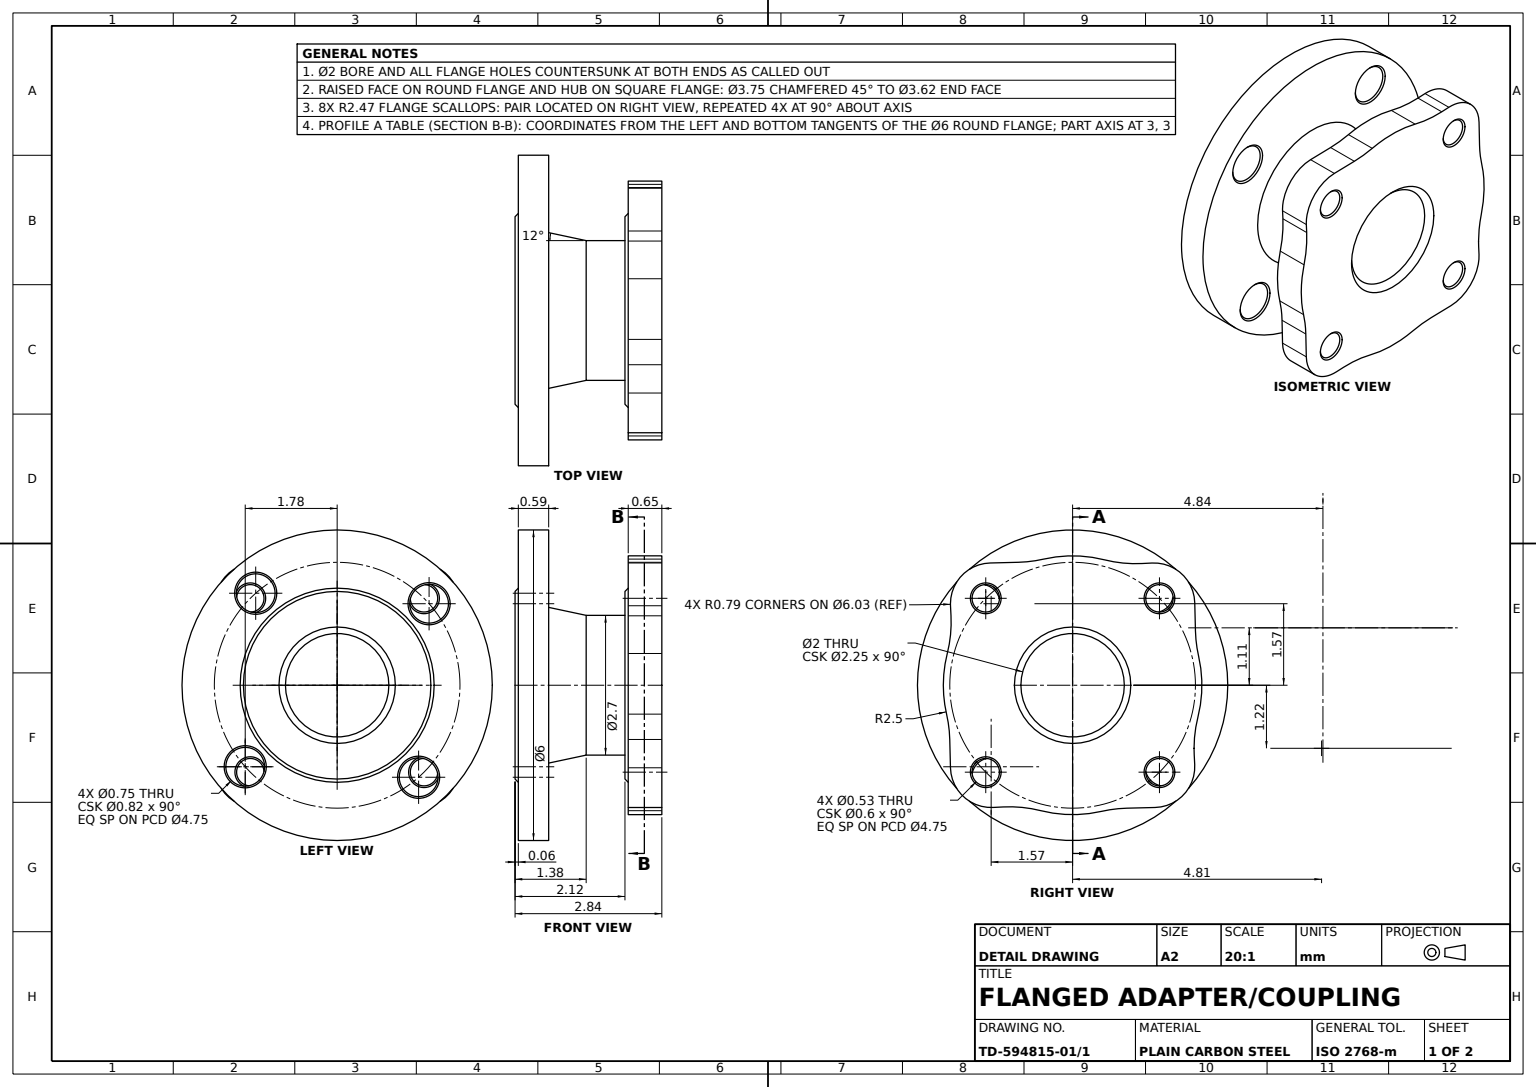
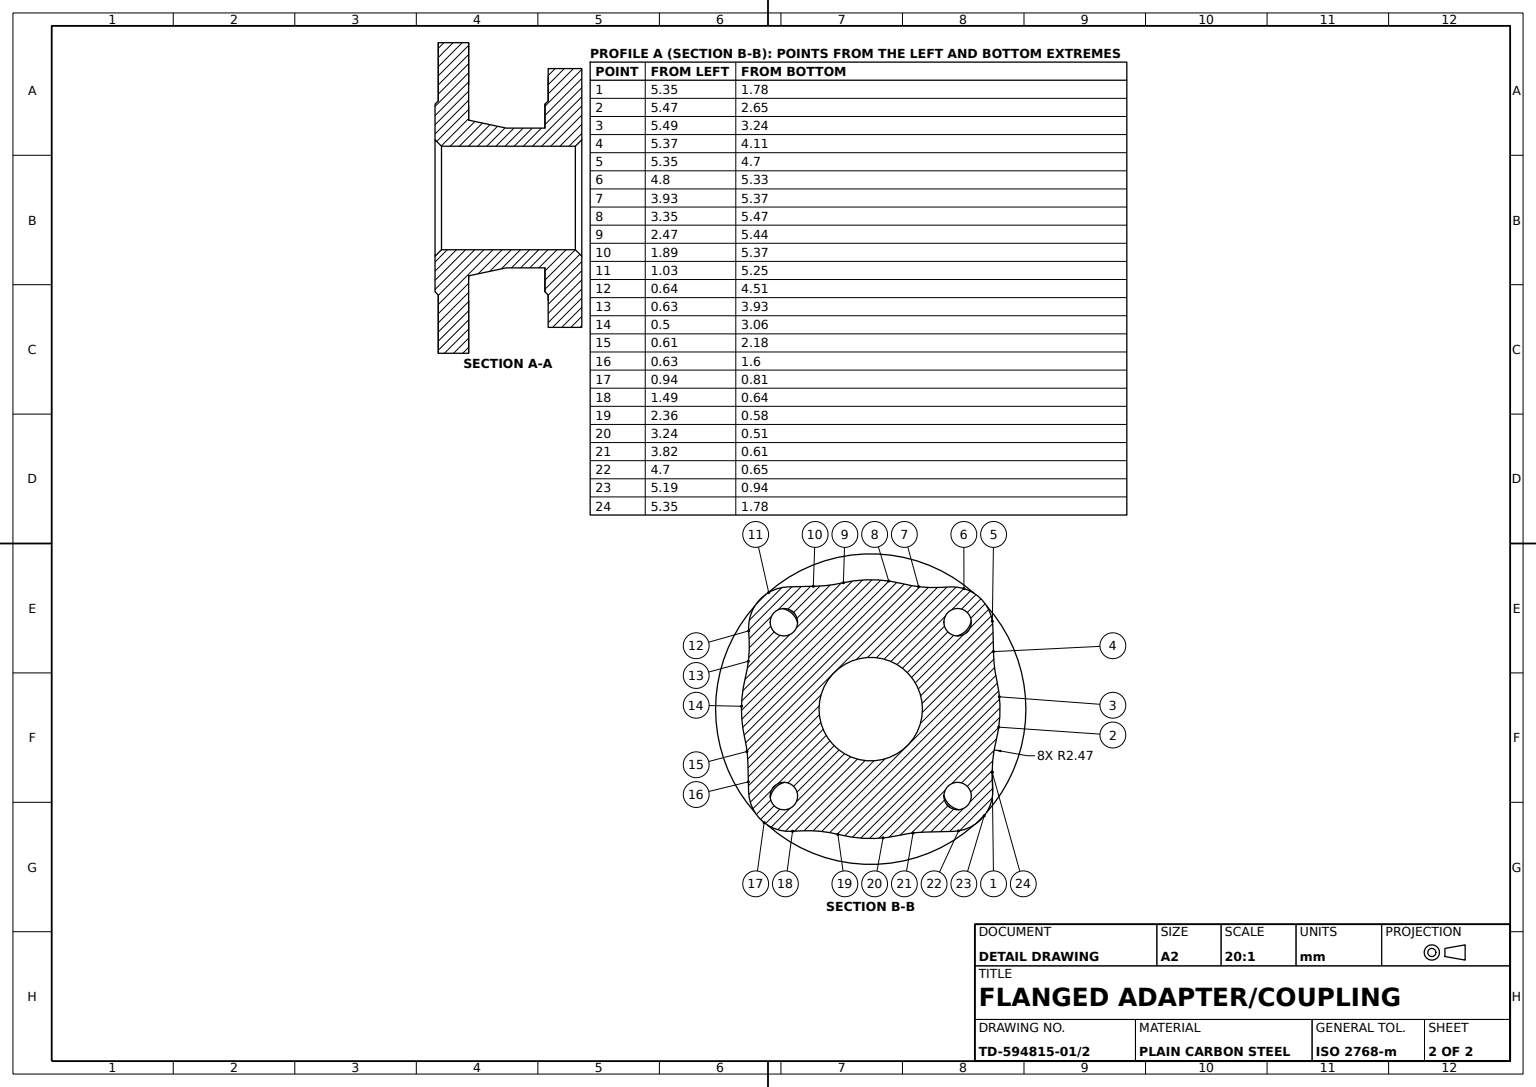
solid
v1 (2.838,0.558304,-2.436862)
v2 (2.838,1.047699,-2.375349)
e1 v1 v2 CIRCLE(AX(P(2.838,1.108969,-4.840385),D(-1,0,0),D(0,0,-1)),2.465797)
v3 (2.188,0.558304,-2.436862)
e2 v1 v3 LINE
v4 (2.188,1.047699,-2.375349)
e3 v3 v4 CIRCLE(AX(P(2.188,1.108969,-4.840385),D(-1,0,0),D(0,0,-1)),2.465797)
e4 v2 v4 LINE
face CYL(AX(P(2.838,1.108969,-4.840385),D(-1,0,0),D(0,0,1)),2.465797) rev [-e1 e2 e3 -e4]
v5 (0.6175,-1.777639,1.95)
v6 (0.65,-1.777639,1.9825)
e5 v5 v6 LINE
v7 (0.65,-1.777639,1.1675)
e6 v7 v6 CIRCLE(AX(P(0.65,-1.777639,1.575),D(-1,0,0),D(0,0,1)),0.4075)
v8 (0.6175,-1.777639,1.2)
e7 v8 v7 LINE
e8 v5 v8 CIRCLE(AX(P(0.6175,-1.777639,1.575),D(1,0,0),D(0,0,1)),0.375)
face CONE(AX(P(0.65,-1.777639,1.575),D(1,0,0),D(0,0,-1)),0.4075,0.785398163) rev [e5 -e6 -e7 -e8]
v9 (2.188,0,1.875)
v10 (2.188,0,-1.875)
e9 v9 v10 CIRCLE(AX(P(2.188,0,0),D(-1,0,0),D(0,0,1)),1.875)
v11 (2.125,0,-1.812)
e10 v11 v10 LINE
v12 (2.125,0,1.812)
e11 v12 v11 CIRCLE(AX(P(2.125,0,0),D(-1,0,0),D(0,0,1)),1.812)
e12 v12 v9 LINE
face CONE(AX(P(2.188,0,0),D(1,0,0),D(0,0,-1)),1.875,0.785398163) [e9 -e10 -e11 e12]
v13 (2.8055,-1.679379,1.414379)
v14 (2.8055,-1.679379,1.944379)
e13 v13 v14 CIRCLE(AX(P(2.8055,-1.679379,1.679379),D(1,0,0),D(0,0,-1)),0.265)
v15 (2.838,-1.679379,1.381879)
e14 v13 v15 LINE
v16 (2.838,-1.679379,1.976879)
e15 v16 v15 CIRCLE(AX(P(2.838,-1.679379,1.679379),D(-1,0,0),D(0,0,-1)),0.2975)
e16 v14 v16 LINE
face CONE(AX(P(2.8055,-1.679379,1.679379),D(1,0,0),D(0,0,-1)),0.265,0.785398163) rev [-e13 e14 -e15 -e16]
v17 (2.2205,-1.679379,-1.944379)
v18 (2.2205,-1.679379,-1.414379)
e17 v17 v18 CIRCLE(AX(P(2.2205,-1.679379,-1.679379),D(-1,0,0),D(0,0,-1)),0.265)
v19 (2.188,-1.679379,-1.976879)
e18 v17 v19 LINE
v20 (2.188,-1.679379,-1.381879)
e19 v20 v19 CIRCLE(AX(P(2.188,-1.679379,-1.679379),D(1,0,0),D(0,0,-1)),0.2975)
e20 v18 v20 LINE
face CONE(AX(P(2.188,-1.679379,-1.679379),D(-1,0,0),D(0,0,1)),0.2975,0.785398163) rev [-e17 e18 -e19 -e20]
v21 (0.0955,-1.777639,1.2)
v22 (0.063,-1.777639,1.1675)
e21 v21 v22 LINE
v23 (0.063,-1.777639,1.9825)
e22 v23 v22 CIRCLE(AX(P(0.063,-1.777639,1.575),D(1,0,0),D(0,0,-1)),0.4075)
v24 (0.0955,-1.777639,1.95)
e23 v24 v23 LINE
e24 v21 v24 CIRCLE(AX(P(0.0955,-1.777639,1.575),D(-1,0,0),D(0,0,-1)),0.375)
face CONE(AX(P(0.0955,-1.777639,1.575),D(-1,0,0),D(0,0,1)),0.375,0.785398163) rev [e21 -e22 -e23 -e24]
v25 (0.6175,-1.575,-1.402639)
v26 (0.65,-1.575,-1.370139)
e25 v25 v26 LINE
v27 (0.65,-1.575,-2.185139)
e26 v27 v26 CIRCLE(AX(P(0.65,-1.575,-1.777639),D(-1,0,0),D(0,0,1)),0.4075)
v28 (0.6175,-1.575,-2.152639)
e27 v28 v27 LINE
e28 v25 v28 CIRCLE(AX(P(0.6175,-1.575,-1.777639),D(1,0,0),D(0,0,1)),0.375)
face CONE(AX(P(0.65,-1.575,-1.777639),D(1,0,0),D(0,0,-1)),0.4075,0.785398163) rev [e25 -e26 -e27 -e28]
v29 (2.8055,1.679379,-1.414379)
v30 (2.838,1.679379,-1.381879)
e29 v29 v30 LINE
v31 (2.8055,1.679379,-1.944379)
e30 v31 v29 CIRCLE(AX(P(2.8055,1.679379,-1.679379),D(1,0,0),D(0,0,-1)),0.265)
v32 (2.838,1.679379,-1.976879)
e31 v31 v32 LINE
e32 v30 v32 CIRCLE(AX(P(2.838,1.679379,-1.679379),D(-1,0,0),D(0,0,-1)),0.2975)
face CONE(AX(P(2.8055,1.679379,-1.679379),D(1,0,0),D(0,0,-1)),0.265,0.785398163) rev [-e29 -e30 e31 -e32]
e33 v11 v12 CIRCLE(AX(P(2.125,0,0),D(-1,0,0),D(0,0,1)),1.812)
v33 (2.125,0,1.35)
v34 (2.125,0,-1.35)
e34 v33 v34 CIRCLE(AX(P(2.125,0,0),D(-1,0,0),D(0,0,1)),1.35)
e35 v34 v33 CIRCLE(AX(P(2.125,0,0),D(-1,0,0),D(0,0,1)),1.35)
face PLANE(AX(P(2.125,1.35,0),D(1,0,0),D(0,0,-1))) rev [e11 e33] [-e34 -e35]
v35 (2.713,0,1)
v36 (2.713,0,-1)
e36 v35 v36 CIRCLE(AX(P(2.713,0,0),D(1,0,0),D(0,0,-1)),1)
v37 (0.125,0,-1)
e37 v36 v37 LINE
v38 (0.125,0,1)
e38 v37 v38 CIRCLE(AX(P(0.125,0,0),D(-1,0,0),D(0,0,-1)),1)
e39 v35 v38 LINE
face CYL(AX(P(0,0,0),D(-1,0,0),D(0,0,1)),1) rev [e36 e37 e38 -e39]
v39 (1.375,0,-1.35)
v40 (1.375,0,1.35)
e40 v39 v40 CIRCLE(AX(P(1.375,0,0),D(-1,0,0),D(0,0,1)),1.35)
e41 v34 v39 LINE
e42 v33 v40 LINE
face CYL(AX(P(0,0,0),D(-1,0,0),D(0,0,1)),1.35) [-e40 -e41 e35 e42]
v41 (2.838,-2.375349,-1.047699)
v42 (2.188,-2.375349,-1.047699)
e43 v41 v42 LINE
v43 (2.188,-2.361757,-1.594555)
e44 v42 v43 LINE
v44 (2.838,-2.361757,-1.594555)
e45 v44 v43 LINE
e46 v41 v44 LINE
face PLANE(AX(P(2.838,-2.361757,-1.594555),D(0,0.999691244,0.024847874),D(0,-0.024847874,0.999691244))) rev [e43 e44 -e45 -e46]
v45 (0.6175,1.575,2.152639)
v46 (0.0955,1.575,2.152639)
e47 v45 v46 LINE
v47 (0.6175,1.575,1.402639)
e48 v45 v47 CIRCLE(AX(P(0.6175,1.575,1.777639),D(1,0,0),D(0,0,1)),0.375)
v48 (0.0955,1.575,1.402639)
e49 v47 v48 LINE
e50 v48 v46 CIRCLE(AX(P(0.0955,1.575,1.777639),D(-1,0,0),D(0,0,-1)),0.375)
face CYL(AX(P(0.713,1.575,1.777639),D(-1,0,0),D(0,0,1)),0.375) rev [-e47 e48 e49 e50]
e51 v8 v21 LINE
e52 v8 v5 CIRCLE(AX(P(0.6175,-1.777639,1.575),D(1,0,0),D(0,0,1)),0.375)
e53 v5 v24 LINE
e54 v24 v21 CIRCLE(AX(P(0.0955,-1.777639,1.575),D(-1,0,0),D(0,0,-1)),0.375)
face CYL(AX(P(0.713,-1.777639,1.575),D(-1,0,0),D(0,0,1)),0.375) rev [-e51 e52 e53 e54]
v49 (0.65,0,3)
v50 (0.65,0,-3)
e55 v49 v50 CIRCLE(AX(P(0.65,0,0),D(-1,0,0),D(0,0,1)),3)
v51 (0.063,0,-3)
e56 v50 v51 LINE
v52 (0.063,0,3)
e57 v52 v51 CIRCLE(AX(P(0.063,0,0),D(-1,0,0),D(0,0,1)),3)
e58 v49 v52 LINE
face CYL(AX(P(0,0,0),D(-1,0,0),D(0,0,1)),3) [e55 e56 -e57 -e58]
v53 (2.188,-2.436862,-0.558304)
e59 v53 v42 CIRCLE(AX(P(2.188,-4.840385,-1.108969),D(-1,0,0),D(0,0,-1)),2.465797)
v54 (2.838,-2.436862,-0.558304)
e60 v54 v41 CIRCLE(AX(P(2.838,-4.840385,-1.108969),D(-1,0,0),D(0,0,-1)),2.465797)
e61 v54 v53 LINE
face CYL(AX(P(2.838,-4.840385,-1.108969),D(-1,0,0),D(0,0,1)),2.465797) rev [e59 -e43 -e60 e61]
e62 v10 v9 CIRCLE(AX(P(2.188,0,0),D(-1,0,0),D(0,0,1)),1.875)
face CONE(AX(P(2.188,0,0),D(1,0,0),D(0,0,-1)),1.875,0.785398163) [e10 e62 -e12 -e33]
v55 (2.838,0,1.125)
e63 v35 v55 LINE
v56 (2.838,0,-1.125)
e64 v56 v55 CIRCLE(AX(P(2.838,0,0),D(-1,0,0),D(0,0,-1)),1.125)
e65 v36 v56 LINE
face CONE(AX(P(2.713,0,0),D(1,0,0),D(0,0,-1)),1,0.785398163) rev [-e36 e63 -e64 -e65]
v57 (0.063,1.777639,-1.9825)
v58 (0.063,1.777639,-1.1675)
e66 v57 v58 CIRCLE(AX(P(0.063,1.777639,-1.575),D(1,0,0),D(0,0,-1)),0.4075)
v59 (0.0955,1.777639,-1.95)
e67 v59 v57 LINE
v60 (0.0955,1.777639,-1.2)
e68 v60 v59 CIRCLE(AX(P(0.0955,1.777639,-1.575),D(-1,0,0),D(0,0,-1)),0.375)
e69 v60 v58 LINE
face CONE(AX(P(0.0955,1.777639,-1.575),D(-1,0,0),D(0,0,1)),0.375,0.785398163) rev [-e66 -e67 -e68 e69]
v61 (2.2205,1.679379,1.414379)
v62 (2.2205,1.679379,1.944379)
e70 v61 v62 CIRCLE(AX(P(2.2205,1.679379,1.679379),D(-1,0,0),D(0,0,-1)),0.265)
v63 (2.188,1.679379,1.381879)
e71 v61 v63 LINE
v64 (2.188,1.679379,1.976879)
e72 v64 v63 CIRCLE(AX(P(2.188,1.679379,1.679379),D(1,0,0),D(0,0,-1)),0.2975)
e73 v62 v64 LINE
face CONE(AX(P(2.188,1.679379,1.679379),D(-1,0,0),D(0,0,1)),0.2975,0.785398163) rev [-e70 e71 -e72 -e73]
v65 (0.063,1.575,2.185139)
e74 v46 v65 LINE
v66 (0.063,1.575,1.370139)
e75 v66 v65 CIRCLE(AX(P(0.063,1.575,1.777639),D(1,0,0),D(0,0,-1)),0.4075)
e76 v48 v66 LINE
e77 v46 v48 CIRCLE(AX(P(0.0955,1.575,1.777639),D(-1,0,0),D(0,0,-1)),0.375)
face CONE(AX(P(0.0955,1.575,1.777639),D(-1,0,0),D(0,0,1)),0.375,0.785398163) rev [e74 -e75 -e76 -e77]
e78 v62 v61 CIRCLE(AX(P(2.2205,1.679379,1.679379),D(-1,0,0),D(0,0,-1)),0.265)
e79 v63 v64 CIRCLE(AX(P(2.188,1.679379,1.679379),D(1,0,0),D(0,0,-1)),0.2975)
face CONE(AX(P(2.188,1.679379,1.679379),D(-1,0,0),D(0,0,1)),0.2975,0.785398163) rev [-e78 e73 -e79 -e71]
v67 (2.2205,1.679379,-1.944379)
e80 v31 v67 LINE
v68 (2.2205,1.679379,-1.414379)
e81 v67 v68 CIRCLE(AX(P(2.2205,1.679379,-1.679379),D(-1,0,0),D(0,0,-1)),0.265)
e82 v29 v68 LINE
e83 v29 v31 CIRCLE(AX(P(2.8055,1.679379,-1.679379),D(1,0,0),D(0,0,-1)),0.265)
face CYL(AX(P(2.838,1.679379,-1.679379),D(-1,0,0),D(0,0,1)),0.265) rev [e80 e81 -e82 e83]
v69 (2.188,1.679379,-1.381879)
e84 v68 v69 LINE
v70 (2.188,1.679379,-1.976879)
e85 v70 v69 CIRCLE(AX(P(2.188,1.679379,-1.679379),D(1,0,0),D(0,0,-1)),0.2975)
e86 v67 v70 LINE
e87 v68 v67 CIRCLE(AX(P(2.2205,1.679379,-1.679379),D(-1,0,0),D(0,0,-1)),0.265)
face CONE(AX(P(2.188,1.679379,-1.679379),D(-1,0,0),D(0,0,1)),0.2975,0.785398163) rev [e84 -e85 -e86 -e87]
v71 (0,0,1.125)
e88 v38 v71 LINE
v72 (0,0,-1.125)
e89 v72 v71 CIRCLE(AX(P(0,0,0),D(1,0,0),D(0,0,-1)),1.125)
e90 v37 v72 LINE
e91 v38 v37 CIRCLE(AX(P(0.125,0,0),D(-1,0,0),D(0,0,-1)),1)
face CONE(AX(P(0.125,0,0),D(-1,0,0),D(0,0,1)),1,0.785398163) rev [e88 -e89 -e90 -e91]
v73 (2.8055,-1.679379,-1.414379)
e92 v73 v18 LINE
e93 v18 v17 CIRCLE(AX(P(2.2205,-1.679379,-1.679379),D(-1,0,0),D(0,0,-1)),0.265)
v74 (2.8055,-1.679379,-1.944379)
e94 v74 v17 LINE
e95 v74 v73 CIRCLE(AX(P(2.8055,-1.679379,-1.679379),D(1,0,0),D(0,0,-1)),0.265)
face CYL(AX(P(2.838,-1.679379,-1.679379),D(-1,0,0),D(0,0,1)),0.265) rev [e92 e93 -e94 e95]
e96 v69 v70 CIRCLE(AX(P(2.188,1.679379,-1.679379),D(1,0,0),D(0,0,-1)),0.2975)
v75 (2.188,-1.679379,1.381879)
v76 (2.188,-1.679379,1.976879)
e97 v75 v76 CIRCLE(AX(P(2.188,-1.679379,1.679379),D(1,0,0),D(0,0,-1)),0.2975)
e98 v76 v75 CIRCLE(AX(P(2.188,-1.679379,1.679379),D(1,0,0),D(0,0,-1)),0.2975)
e99 v19 v20 CIRCLE(AX(P(2.188,-1.679379,-1.679379),D(1,0,0),D(0,0,-1)),0.2975)
v77 (2.188,-1.218309,-2.348231)
v78 (2.188,-0.61335,-2.423593)
e100 v77 v78 CIRCLE(AX(P(2.188,-1.218309,-4.814028),D(-1,0,0),D(0,0,1)),2.465797)
v79 (2.188,-1.341424,-2.351306)
e101 v79 v77 CIRCLE(AX(P(2.188,-1.218309,-4.814028),D(-1,0,0),D(0,0,1)),2.465797)
v80 (2.188,-1.535706,-2.361018)
e102 v80 v79 LINE
e103 v43 v80 CIRCLE(AX(P(2.188,-1.575,-1.575),D(1,0,0),D(0,0,-1)),0.787)
v81 (2.188,-2.423593,0.61335)
e104 v81 v53 CIRCLE(AX(P(2.188,0,0),D(1,0,0),D(0,0,-1)),2.5)
v82 (2.188,-2.351306,1.341424)
e105 v82 v81 CIRCLE(AX(P(2.188,-4.814028,1.218309),D(-1,0,0),D(0,0,1)),2.465797)
v83 (2.188,-2.361018,1.535706)
e106 v83 v82 LINE
v84 (2.188,-1.594555,2.361757)
e107 v84 v83 CIRCLE(AX(P(2.188,-1.575,1.575),D(1,0,0),D(0,0,-1)),0.787)
v85 (2.188,-1.047699,2.375349)
e108 v85 v84 LINE
v86 (2.188,-0.558304,2.436862)
e109 v86 v85 CIRCLE(AX(P(2.188,-1.108969,4.840385),D(-1,0,0),D(0,0,-1)),2.465797)
v87 (2.188,0,2.5)
e110 v87 v86 CIRCLE(AX(P(2.188,0,0),D(1,0,0),D(0,0,-1)),2.5)
v88 (2.188,0.61335,2.423593)
e111 v88 v87 CIRCLE(AX(P(2.188,0,0),D(1,0,0),D(0,0,-1)),2.5)
v89 (2.188,1.341424,2.351306)
e112 v89 v88 CIRCLE(AX(P(2.188,1.218309,4.814028),D(-1,0,0),D(0,0,1)),2.465797)
v90 (2.188,1.535706,2.361018)
e113 v90 v89 LINE
v91 (2.188,1.575,2.362)
e114 v91 v90 CIRCLE(AX(P(2.188,1.575,1.575),D(1,0,0),D(0,0,-1)),0.787)
v92 (2.188,2.361757,1.594555)
e115 v92 v91 CIRCLE(AX(P(2.188,1.575,1.575),D(1,0,0),D(0,0,-1)),0.787)
v93 (2.188,2.375349,1.047699)
e116 v93 v92 LINE
v94 (2.188,2.436862,0.558304)
e117 v94 v93 CIRCLE(AX(P(2.188,4.840385,1.108969),D(-1,0,0),D(0,0,1)),2.465797)
v95 (2.188,2.423593,-0.61335)
e118 v95 v94 CIRCLE(AX(P(2.188,0,0),D(1,0,0),D(0,0,-1)),2.5)
v96 (2.188,2.351306,-1.341424)
e119 v96 v95 CIRCLE(AX(P(2.188,4.814028,-1.218309),D(-1,0,0),D(0,0,1)),2.465797)
v97 (2.188,2.361018,-1.535706)
e120 v97 v96 LINE
v98 (2.188,1.594555,-2.361757)
e121 v98 v97 CIRCLE(AX(P(2.188,1.575,-1.575),D(1,0,0),D(0,0,-1)),0.787)
e122 v4 v98 LINE
e123 v78 v3 CIRCLE(AX(P(2.188,0,0),D(1,0,0),D(0,0,-1)),2.5)
face PLANE(AX(P(2.188,1.575,1.575),D(1,0,0),D(0,0,-1))) rev [e96 e85] [e97 e98] [e19 e99] [-e62 -e9] [e79 e72] [-e100 -e101 -e102 -e103 -e44 -e59 -e104 -e105 -e106 -e107 -e108 -e109 -e110 -e111 -e112 -e113 -e114 -e115 -e116 -e117 -e118 -e119 -e120 -e121 -e122 -e3 -e123]
v99 (2.838,-0.61335,-2.423593)
e124 v99 v78 LINE
v100 (2.838,-1.218309,-2.348231)
e125 v100 v99 CIRCLE(AX(P(2.838,-1.218309,-4.814028),D(-1,0,0),D(0,0,1)),2.465797)
e126 v100 v77 LINE
face CYL(AX(P(2.838,-1.218309,-4.814028),D(-1,0,0),D(0,0,1)),2.465797) rev [e100 -e124 -e125 e126]
v101 (2.838,-1.535706,-2.361018)
e127 v101 v80 LINE
e128 v44 v101 CIRCLE(AX(P(2.838,-1.575,-1.575),D(1,0,0),D(0,0,-1)),0.787)
face CYL(AX(P(2.838,-1.575,-1.575),D(-1,0,0),D(0,0,1)),0.787) [-e127 -e128 e45 e103]
v102 (0.6175,1.777639,-1.95)
v103 (0.6175,1.777639,-1.2)
e129 v102 v103 CIRCLE(AX(P(0.6175,1.777639,-1.575),D(1,0,0),D(0,0,1)),0.375)
v104 (0.65,1.777639,-1.9825)
e130 v102 v104 LINE
v105 (0.65,1.777639,-1.1675)
e131 v105 v104 CIRCLE(AX(P(0.65,1.777639,-1.575),D(-1,0,0),D(0,0,1)),0.4075)
e132 v103 v105 LINE
face CONE(AX(P(0.65,1.777639,-1.575),D(1,0,0),D(0,0,-1)),0.4075,0.785398163) rev [-e129 e130 -e131 -e132]
e133 v65 v66 CIRCLE(AX(P(0.063,1.575,1.777639),D(1,0,0),D(0,0,-1)),0.4075)
e134 v22 v23 CIRCLE(AX(P(0.063,-1.777639,1.575),D(1,0,0),D(0,0,-1)),0.4075)
v106 (0.063,0,-1.8755)
v107 (0.063,0,1.8755)
e135 v106 v107 CIRCLE(AX(P(0.063,0,0),D(-1,0,0),D(0,0,1)),1.8755)
e136 v107 v106 CIRCLE(AX(P(0.063,0,0),D(-1,0,0),D(0,0,1)),1.8755)
e137 v58 v57 CIRCLE(AX(P(0.063,1.777639,-1.575),D(1,0,0),D(0,0,-1)),0.4075)
e138 v51 v52 CIRCLE(AX(P(0.063,0,0),D(-1,0,0),D(0,0,1)),3)
v108 (0.063,-1.575,-2.185139)
v109 (0.063,-1.575,-1.370139)
e139 v108 v109 CIRCLE(AX(P(0.063,-1.575,-1.777639),D(1,0,0),D(0,0,-1)),0.4075)
e140 v109 v108 CIRCLE(AX(P(0.063,-1.575,-1.777639),D(1,0,0),D(0,0,-1)),0.4075)
face PLANE(AX(P(0.063,1.8755,0),D(1,0,0),D(0,0,-1))) rev [e133 e75] [e22 e134] [-e135 -e136] [e137 e66] [e138 e57] [e139 e140]
e141 v103 v102 CIRCLE(AX(P(0.6175,1.777639,-1.575),D(1,0,0),D(0,0,1)),0.375)
e142 v104 v105 CIRCLE(AX(P(0.65,1.777639,-1.575),D(-1,0,0),D(0,0,1)),0.4075)
face CONE(AX(P(0.65,1.777639,-1.575),D(1,0,0),D(0,0,-1)),0.4075,0.785398163) rev [-e141 e132 -e142 -e130]
v110 (2.8055,1.679379,1.944379)
e143 v110 v62 LINE
v111 (2.8055,1.679379,1.414379)
e144 v111 v61 LINE
e145 v111 v110 CIRCLE(AX(P(2.8055,1.679379,1.679379),D(1,0,0),D(0,0,-1)),0.265)
face CYL(AX(P(2.838,1.679379,1.679379),D(-1,0,0),D(0,0,1)),0.265) rev [e143 e78 -e144 e145]
v112 (0.0955,-1.575,-1.402639)
v113 (0.0955,-1.575,-2.152639)
e146 v112 v113 CIRCLE(AX(P(0.0955,-1.575,-1.777639),D(-1,0,0),D(0,0,-1)),0.375)
e147 v28 v113 LINE
e148 v28 v25 CIRCLE(AX(P(0.6175,-1.575,-1.777639),D(1,0,0),D(0,0,1)),0.375)
e149 v25 v112 LINE
face CYL(AX(P(0.713,-1.575,-1.777639),D(-1,0,0),D(0,0,1)),0.375) rev [e146 -e147 e148 e149]
e150 v26 v27 CIRCLE(AX(P(0.65,-1.575,-1.777639),D(-1,0,0),D(0,0,1)),0.4075)
face CONE(AX(P(0.65,-1.575,-1.777639),D(1,0,0),D(0,0,-1)),0.4075,0.785398163) rev [e27 -e150 -e25 -e148]
face CYL(AX(P(2.838,1.679379,-1.679379),D(-1,0,0),D(0,0,1)),0.265) rev [-e80 e30 e82 e87]
v114 (2.838,-0.558304,2.436862)
e151 v114 v86 LINE
v115 (2.838,0,2.5)
e152 v115 v114 CIRCLE(AX(P(2.838,0,0),D(1,0,0),D(0,0,-1)),2.5)
e153 v115 v87 LINE
face CYL(AX(P(2.838,0,0),D(-1,0,0),D(0,0,1)),2.5) [-e151 -e152 e153 e110]
e154 v32 v30 CIRCLE(AX(P(2.838,1.679379,-1.679379),D(-1,0,0),D(0,0,-1)),0.2975)
face CONE(AX(P(2.8055,1.679379,-1.679379),D(1,0,0),D(0,0,-1)),0.265,0.785398163) rev [-e83 e29 -e154 -e31]
face CONE(AX(P(2.188,-1.679379,-1.679379),D(-1,0,0),D(0,0,1)),0.2975,0.785398163) rev [-e18 -e93 e20 -e99]
v116 (2.2205,-1.679379,1.414379)
e155 v13 v116 LINE
v117 (2.2205,-1.679379,1.944379)
e156 v116 v117 CIRCLE(AX(P(2.2205,-1.679379,1.679379),D(-1,0,0),D(0,0,-1)),0.265)
e157 v14 v117 LINE
e158 v14 v13 CIRCLE(AX(P(2.8055,-1.679379,1.679379),D(1,0,0),D(0,0,-1)),0.265)
face CYL(AX(P(2.838,-1.679379,1.679379),D(-1,0,0),D(0,0,1)),0.265) rev [e155 e156 -e157 e158]
e159 v117 v76 LINE
e160 v116 v75 LINE
e161 v117 v116 CIRCLE(AX(P(2.2205,-1.679379,1.679379),D(-1,0,0),D(0,0,-1)),0.265)
face CONE(AX(P(2.188,-1.679379,1.679379),D(-1,0,0),D(0,0,1)),0.2975,0.785398163) rev [e159 -e97 -e160 -e161]
e162 v47 v45 CIRCLE(AX(P(0.6175,1.575,1.777639),D(1,0,0),D(0,0,1)),0.375)
face CYL(AX(P(0.713,1.575,1.777639),D(-1,0,0),D(0,0,1)),0.375) rev [e77 -e49 e162 e47]
v118 (2.838,-1.341424,-2.351306)
e163 v118 v79 LINE
e164 v101 v118 LINE
face PLANE(AX(P(2.838,-1.535706,-2.361018),D(0,-0.049928951,0.998752772),D(0,-0.998752772,-0.049928951))) rev [-e163 -e164 e127 e102]
v119 (0.65,1.575,1.370139)
e165 v47 v119 LINE
v120 (0.65,1.575,2.185139)
e166 v120 v119 CIRCLE(AX(P(0.65,1.575,1.777639),D(-1,0,0),D(0,0,1)),0.4075)
e167 v45 v120 LINE
face CONE(AX(P(0.65,1.575,1.777639),D(1,0,0),D(0,0,-1)),0.4075,0.785398163) rev [-e162 e165 -e166 -e167]
e168 v6 v7 CIRCLE(AX(P(0.65,-1.777639,1.575),D(-1,0,0),D(0,0,1)),0.4075)
e169 v50 v49 CIRCLE(AX(P(0.65,0,0),D(-1,0,0),D(0,0,1)),3)
v121 (0.65,0,-1.504104)
v122 (0.65,0,1.504104)
e170 v121 v122 CIRCLE(AX(P(0.65,0,0),D(-1,0,0),D(0,0,1)),1.504104)
e171 v122 v121 CIRCLE(AX(P(0.65,0,0),D(-1,0,0),D(0,0,1)),1.504104)
e172 v119 v120 CIRCLE(AX(P(0.65,1.575,1.777639),D(-1,0,0),D(0,0,1)),0.4075)
face PLANE(AX(P(0.65,3,0),D(-1,0,0),D(0,0,1))) rev [e6 e168] [-e169 -e55] [e170 e171] [e172 e166] [e150 e26] [e142 e131]
face CONE(AX(P(0.0955,1.575,1.777639),D(-1,0,0),D(0,0,1)),0.375,0.785398163) rev [-e50 e76 -e133 -e74]
v123 (2.838,1.594555,-2.361757)
e173 v123 v98 LINE
e174 v2 v123 LINE
face PLANE(AX(P(2.838,1.594555,-2.361757),D(0,-0.024847874,0.999691244),D(0,-0.999691244,-0.024847874))) rev [e4 e122 -e173 -e174]
v124 (2.838,-1.679379,-1.976879)
v125 (2.838,-1.679379,-1.381879)
e175 v124 v125 CIRCLE(AX(P(2.838,-1.679379,-1.679379),D(-1,0,0),D(0,0,-1)),0.2975)
e176 v74 v124 LINE
e177 v73 v74 CIRCLE(AX(P(2.8055,-1.679379,-1.679379),D(1,0,0),D(0,0,-1)),0.265)
e178 v73 v125 LINE
face CONE(AX(P(2.8055,-1.679379,-1.679379),D(1,0,0),D(0,0,-1)),0.265,0.785398163) rev [-e175 -e176 -e177 e178]
e179 v36 v35 CIRCLE(AX(P(2.713,0,0),D(1,0,0),D(0,0,-1)),1)
e180 v55 v56 CIRCLE(AX(P(2.838,0,0),D(-1,0,0),D(0,0,-1)),1.125)
face CONE(AX(P(2.713,0,0),D(1,0,0),D(0,0,-1)),1,0.785398163) rev [-e179 e65 -e180 -e63]
v126 (2.838,2.423593,-0.61335)
v127 (2.838,2.436862,0.558304)
e181 v126 v127 CIRCLE(AX(P(2.838,0,0),D(1,0,0),D(0,0,-1)),2.5)
e182 v126 v95 LINE
e183 v127 v94 LINE
face CYL(AX(P(2.838,0,0),D(-1,0,0),D(0,0,1)),2.5) [-e181 e182 e118 -e183]
v128 (2.838,2.361018,-1.535706)
e184 v128 v97 LINE
e185 v123 v128 CIRCLE(AX(P(2.838,1.575,-1.575),D(1,0,0),D(0,0,-1)),0.787)
face CYL(AX(P(2.838,1.575,-1.575),D(-1,0,0),D(0,0,1)),0.787) [e121 -e184 -e185 e173]
v129 (2.838,-1.047699,2.375349)
e186 v129 v85 LINE
e187 v114 v129 CIRCLE(AX(P(2.838,-1.108969,4.840385),D(-1,0,0),D(0,0,-1)),2.465797)
face CYL(AX(P(2.838,-1.108969,4.840385),D(-1,0,0),D(0,0,1)),2.465797) rev [e151 e109 -e186 -e187]
v130 (2.838,1.535706,2.361018)
e188 v130 v90 LINE
v131 (2.838,1.575,2.362)
e189 v131 v130 CIRCLE(AX(P(2.838,1.575,1.575),D(1,0,0),D(0,0,-1)),0.787)
e190 v131 v91 LINE
face CYL(AX(P(2.838,1.575,1.575),D(-1,0,0),D(0,0,1)),0.787) [e114 -e188 -e189 e190]
face CYL(AX(P(0.713,-1.777639,1.575),D(-1,0,0),D(0,0,1)),0.375) rev [e51 e24 -e53 e8]
e191 v71 v72 CIRCLE(AX(P(0,0,0),D(1,0,0),D(0,0,-1)),1.125)
v132 (0,0,1.8125)
v133 (0,0,-1.8125)
e192 v132 v133 CIRCLE(AX(P(0,0,0),D(-1,0,0),D(0,0,1)),1.8125)
e193 v133 v132 CIRCLE(AX(P(0,0,0),D(-1,0,0),D(0,0,1)),1.8125)
face PLANE(AX(P(0,1,0),D(1,0,0),D(0,0,-1))) rev [e191 e89] [e192 e193]
e194 v125 v124 CIRCLE(AX(P(2.838,-1.679379,-1.679379),D(-1,0,0),D(0,0,-1)),0.2975)
face CONE(AX(P(2.8055,-1.679379,-1.679379),D(1,0,0),D(0,0,-1)),0.265,0.785398163) rev [-e194 -e178 -e95 e176]
v134 (2.838,1.341424,2.351306)
e195 v134 v89 LINE
e196 v130 v134 LINE
face PLANE(AX(P(2.838,1.535706,2.361018),D(0,0.049928951,-0.998752772),D(0,0.998752772,0.049928951))) rev [e113 -e195 -e196 e188]
face CYL(AX(P(2.838,-1.679379,-1.679379),D(-1,0,0),D(0,0,1)),0.265) rev [-e92 e177 e94 e17]
v135 (2.838,2.351306,-1.341424)
e197 v135 v96 LINE
e198 v135 v126 CIRCLE(AX(P(2.838,4.814028,-1.218309),D(-1,0,0),D(0,0,1)),2.465797)
face CYL(AX(P(2.838,4.814028,-1.218309),D(-1,0,0),D(0,0,1)),2.465797) rev [e197 e119 -e182 -e198]
v136 (2.838,2.375349,1.047699)
e199 v136 v93 LINE
e200 v127 v136 CIRCLE(AX(P(2.838,4.840385,1.108969),D(-1,0,0),D(0,0,1)),2.465797)
face CYL(AX(P(2.838,4.840385,1.108969),D(-1,0,0),D(0,0,1)),2.465797) rev [-e199 -e200 e183 e117]
face CYL(AX(P(0,0,0),D(-1,0,0),D(0,0,1)),3) [e58 -e138 -e56 e169]
e201 v40 v39 CIRCLE(AX(P(1.375,0,0),D(-1,0,0),D(0,0,1)),1.35)
face CYL(AX(P(0,0,0),D(-1,0,0),D(0,0,1)),1.35) [-e201 -e42 e34 e41]
face CONE(AX(P(0.65,-1.777639,1.575),D(1,0,0),D(0,0,-1)),0.4075,0.785398163) rev [-e168 -e5 -e52 e7]
v137 (2.838,-1.594555,2.361757)
e202 v137 v84 LINE
e203 v129 v137 LINE
face PLANE(AX(P(2.838,-1.594555,2.361757),D(0,0.024847874,-0.999691244),D(0,0.999691244,0.024847874))) rev [e186 e108 -e202 -e203]
face CYL(AX(P(2.838,-1.679379,1.679379),D(-1,0,0),D(0,0,1)),0.265) rev [-e155 e13 e157 e161]
v138 (2.838,2.361757,1.594555)
e204 v138 v131 CIRCLE(AX(P(2.838,1.575,1.575),D(1,0,0),D(0,0,-1)),0.787)
v139 (2.838,0.61335,2.423593)
e205 v134 v139 CIRCLE(AX(P(2.838,1.218309,4.814028),D(-1,0,0),D(0,0,1)),2.465797)
e206 v139 v115 CIRCLE(AX(P(2.838,0,0),D(1,0,0),D(0,0,-1)),2.5)
v140 (2.838,-2.361018,1.535706)
e207 v137 v140 CIRCLE(AX(P(2.838,-1.575,1.575),D(1,0,0),D(0,0,-1)),0.787)
v141 (2.838,-2.351306,1.341424)
e208 v140 v141 LINE
v142 (2.838,-2.423593,0.61335)
e209 v141 v142 CIRCLE(AX(P(2.838,-4.814028,1.218309),D(-1,0,0),D(0,0,1)),2.465797)
e210 v142 v54 CIRCLE(AX(P(2.838,0,0),D(1,0,0),D(0,0,-1)),2.5)
e211 v118 v100 CIRCLE(AX(P(2.838,-1.218309,-4.814028),D(-1,0,0),D(0,0,1)),2.465797)
e212 v99 v1 CIRCLE(AX(P(2.838,0,0),D(1,0,0),D(0,0,-1)),2.5)
e213 v128 v135 LINE
e214 v136 v138 LINE
e215 v15 v16 CIRCLE(AX(P(2.838,-1.679379,1.679379),D(-1,0,0),D(0,0,-1)),0.2975)
v143 (2.838,1.679379,1.976879)
v144 (2.838,1.679379,1.381879)
e216 v143 v144 CIRCLE(AX(P(2.838,1.679379,1.679379),D(-1,0,0),D(0,0,-1)),0.2975)
e217 v144 v143 CIRCLE(AX(P(2.838,1.679379,1.679379),D(-1,0,0),D(0,0,-1)),0.2975)
face PLANE(AX(P(2.838,1.575,1.575),D(1,0,0),D(0,0,-1))) [e32 e154] [e64 e180] [e204 e189 e196 e205 e206 e152 e187 e203 e207 e208 e209 e210 e60 e46 e128 e164 e211 e125 e212 e1 e174 e185 e213 e198 e181 e200 e214] [e15 e215] [e175 e194] [e216 e217]
e218 v139 v88 LINE
face CYL(AX(P(2.838,1.218309,4.814028),D(-1,0,0),D(0,0,1)),2.465797) rev [-e218 -e205 e195 e112]
face CYL(AX(P(2.838,0,0),D(-1,0,0),D(0,0,1)),2.5) [-e206 e218 e111 -e153]
e219 v132 v107 LINE
e220 v133 v106 LINE
face CONE(AX(P(0.063,0,0),D(1,0,0),D(0,0,-1)),1.8755,0.785398163) [e135 -e219 -e193 e220]
e221 v40 v122 LINE
e222 v39 v121 LINE
face CONE(AX(P(1.375,0,0),D(-1,0,0),D(0,0,1)),1.35,0.20943951) [e221 -e170 -e222 e40]
e223 v112 v109 LINE
e224 v113 v112 CIRCLE(AX(P(0.0955,-1.575,-1.777639),D(-1,0,0),D(0,0,-1)),0.375)
e225 v113 v108 LINE
face CONE(AX(P(0.0955,-1.575,-1.777639),D(-1,0,0),D(0,0,1)),0.375,0.785398163) rev [-e223 -e224 e225 -e140]
face CONE(AX(P(1.375,0,0),D(-1,0,0),D(0,0,1)),1.35,0.20943951) [e222 -e171 -e221 e201]
e226 v138 v92 LINE
face PLANE(AX(P(2.838,2.361757,1.594555),D(0,-0.999691244,-0.024847874),D(0,0.024847874,-0.999691244))) rev [-e214 e199 e116 -e226]
face CYL(AX(P(0.713,-1.575,-1.777639),D(-1,0,0),D(0,0,1)),0.375) rev [e224 -e149 e28 e147]
e227 v110 v143 LINE
e228 v111 v144 LINE
e229 v110 v111 CIRCLE(AX(P(2.8055,1.679379,1.679379),D(1,0,0),D(0,0,-1)),0.265)
face CONE(AX(P(2.8055,1.679379,1.679379),D(1,0,0),D(0,0,-1)),0.265,0.785398163) rev [e227 -e217 -e228 -e229]
face CYL(AX(P(0,0,0),D(-1,0,0),D(0,0,1)),1) rev [e91 -e37 e179 e39]
e230 v141 v82 LINE
e231 v140 v83 LINE
face PLANE(AX(P(2.838,-2.361018,1.535706),D(0,0.998752772,0.049928951),D(0,-0.049928951,0.998752772))) rev [e106 -e230 -e208 e231]
face CONE(AX(P(0.125,0,0),D(-1,0,0),D(0,0,1)),1,0.785398163) rev [-e88 -e38 e90 -e191]
face CYL(AX(P(2.838,0,0),D(-1,0,0),D(0,0,1)),2.5) [-e212 e124 e123 -e2]
face CONE(AX(P(2.8055,1.679379,1.679379),D(1,0,0),D(0,0,-1)),0.265,0.785398163) rev [-e216 -e227 -e145 e228]
face CYL(AX(P(2.838,-1.218309,-4.814028),D(-1,0,0),D(0,0,1)),2.465797) rev [e163 e101 -e126 -e211]
face CONE(AX(P(2.188,-1.679379,1.679379),D(-1,0,0),D(0,0,1)),0.2975,0.785398163) rev [-e98 -e159 -e156 e160]
face CYL(AX(P(2.838,-1.575,1.575),D(-1,0,0),D(0,0,1)),0.787) [-e207 e202 e107 -e231]
face CONE(AX(P(2.8055,-1.679379,1.679379),D(1,0,0),D(0,0,-1)),0.265,0.785398163) rev [-e215 -e14 -e158 e16]
e232 v142 v81 LINE
face CYL(AX(P(2.838,0,0),D(-1,0,0),D(0,0,1)),2.5) [e232 e104 -e61 -e210]
e233 v59 v60 CIRCLE(AX(P(0.0955,1.777639,-1.575),D(-1,0,0),D(0,0,-1)),0.375)
face CONE(AX(P(0.0955,1.777639,-1.575),D(-1,0,0),D(0,0,1)),0.375,0.785398163) rev [-e69 -e233 e67 -e137]
face PLANE(AX(P(2.838,2.361018,-1.535706),D(0,-0.998752772,-0.049928951),D(0,0.049928951,-0.998752772))) rev [-e197 -e213 e184 e120]
e234 v102 v59 LINE
e235 v103 v60 LINE
face CYL(AX(P(0.713,1.777639,-1.575),D(-1,0,0),D(0,0,1)),0.375) rev [e141 e234 e233 -e235]
face CYL(AX(P(2.838,1.679379,1.679379),D(-1,0,0),D(0,0,1)),0.265) rev [e144 e70 -e143 e229]
face CYL(AX(P(0.713,1.777639,-1.575),D(-1,0,0),D(0,0,1)),0.375) rev [-e234 e129 e235 e68]
face CONE(AX(P(0.063,0,0),D(1,0,0),D(0,0,-1)),1.8755,0.785398163) [e136 -e220 -e192 e219]
face CYL(AX(P(2.838,1.575,1.575),D(-1,0,0),D(0,0,1)),0.787) [-e204 e226 e115 -e190]
face CONE(AX(P(2.188,1.679379,-1.679379),D(-1,0,0),D(0,0,1)),0.2975,0.785398163) rev [-e96 -e84 -e81 e86]
face CYL(AX(P(2.838,-4.814028,1.218309),D(-1,0,0),D(0,0,1)),2.465797) rev [-e232 -e209 e230 e105]
face CONE(AX(P(0.0955,-1.575,-1.777639),D(-1,0,0),D(0,0,1)),0.375,0.785398163) rev [e223 -e139 -e225 -e146]
face CONE(AX(P(0.0955,-1.777639,1.575),D(-1,0,0),D(0,0,1)),0.375,0.785398163) rev [e23 -e134 -e21 -e54]
face CONE(AX(P(0.65,1.575,1.777639),D(1,0,0),D(0,0,-1)),0.4075,0.785398163) rev [-e48 e167 -e172 -e165]
